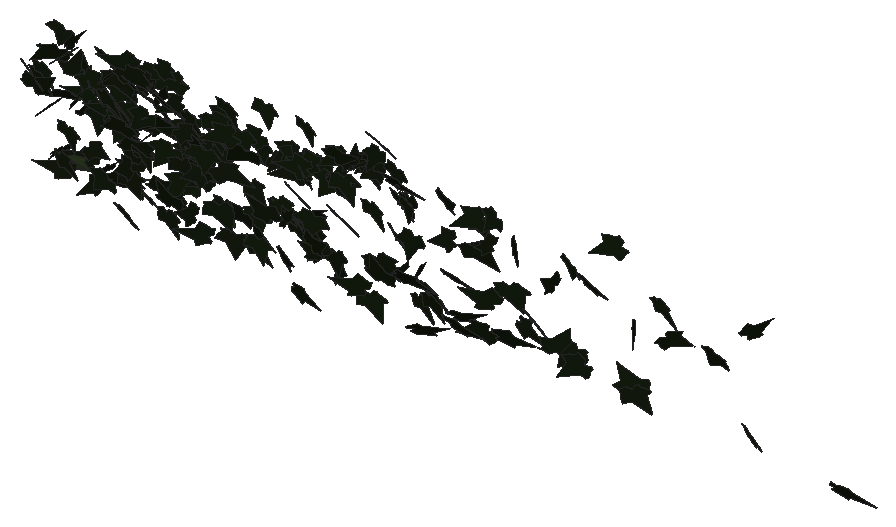
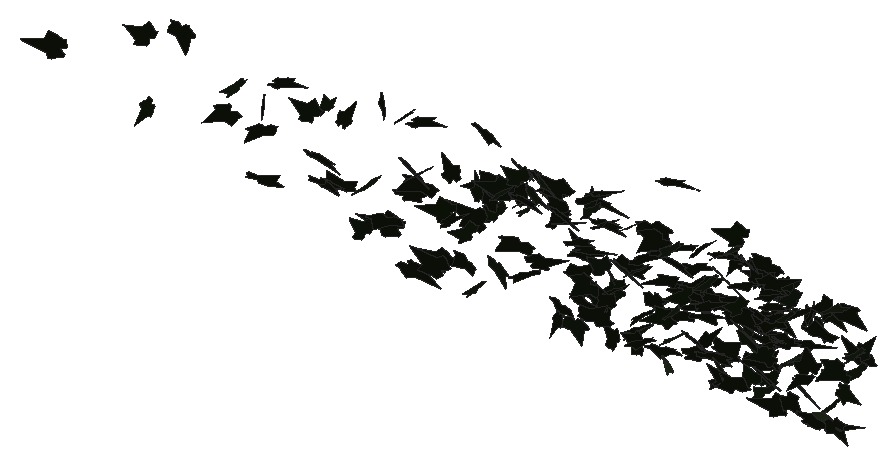
# SketchUp Ruby script. Lengths in millimetres.
U = 1.mm
M = Sketchup.active_model
def pt(a) = Geom::Point3d.new(a.map { |v| v * U })
def face(e, loops, mat)
  f = e.add_face(loops[0].map { |a| pt(a) })
  loops[1..].each { |l| e.add_face(l.map { |a| pt(a) }).erase! }
  f.material = f.back_material = mat if mat
  f
end
# faces: each face lists its corners as indices into pts; further lists are holes
def faces(e, pts, list, mat = nil) = list.each { |f| face(e, (f[0].is_a?(Array) ? f : [f]).map { |l| l.map { |i| pts[i] } }, mat) }
# xy, xz, yz: faces in a plane at the given z, y or x. An outline is a flat list of corners, or four numbers for a rectangle; further outlines are holes
def ring(l) = l.size == 4 ? [[l[0], l[1]], [l[2], l[1]], [l[2], l[3]], [l[0], l[3]]] : l.each_slice(2).to_a
def flat(e, list, mat, &to3) = list.each { |f| face(e, (f[0].is_a?(Array) ? f : [f]).map { |l| ring(l).map { |u, v| to3.(u, v) } }, mat) }
def xy(e, z, list, mat = nil) = flat(e, list, mat) { |x, y| [x, y, z] }
def xz(e, y, list, mat = nil) = flat(e, list, mat) { |x, z| [x, y, z] }
def yz(e, x, list, mat = nil) = flat(e, list, mat) { |y, z| [x, y, z] }
def lines(e, pts, list) = list.each { |a, b| e.add_line(pt(pts[a]), pt(pts[b])) }
# prism: a flat outline (further loops are holes) pulled along v
def prism(e, loops, v, mat = nil)
  f = face(e, loops, mat); d = Geom::Vector3d.new(v.map { |x| x * U })
  f.pushpull(f.normal.samedirection?(d) ? d.length : -d.length)
end
def box(e, o, s, mat = nil) = prism(e, [[o, [o[0] + s[0], o[1], o[2]], [o[0] + s[0], o[1] + s[1], o[2]], [o[0], o[1] + s[1], o[2]]]], [0, 0, s[2]], mat)
def at(x, y, z, deg = 0) = Geom::Transformation.translation(pt([x, y, z])) * Geom::Transformation.rotation(ORIGIN, Z_AXIS, deg.degrees)
def axes(o, x, y, z) = Geom::Transformation.new([*x, 0, *y, 0, *z, 0, *pt(o).to_a, 1])
def part(name) = M.definitions.add(name)
# library, detail: a bought-in or finely detailed component or shape, given as its bounding box
def library(name, o, s) = part(name).tap { |d| box(d.entities, o, s) }
def detail(e, o, s) = box(e.add_group.entities, o, s)
def put(e, d, t, mat = nil) = e.add_instance(d, t).tap { |i| i.material = mat if mat }
def group(e, t, mat = nil) = e.add_group.tap { |g| g.transformation = t; g.material = mat if mat }.entities
root = M.entities
M.materials.add("efeu1").color = [18, 25, 13]
M.materials.add("efeu2").color = [43, 57, 29]
c1 = part("ivyleaf_9")
p = [[39.1,54.8,31.7],[34.5,51.8,30.2],[-5.3,25.2,17.3],[-17.9,28.3,20.9],[-21.6,21.7,17],[-20.2,4.3,5.3],
  [-22.9,-0.3,2.5],[-17.1,-4,-0.6],[-2,-2.1,-1.2],[-0.7,-15.4,-10.1],[16.6,-22.3,-16.7],[21.1,-15.1,-12.5],
  [32.7,-10.7,-11],[46.1,-1.8,-6.6],[30.8,11.2,3.8]]
faces(c1.entities,p,[[0,1,2,3,4,5,6,7,8,9,10,11,12,13,14]],"efeu1")
c2 = part("ivyleaf_10")
p = [[0,12.8,-0.8],[-1.5,51.3,-10.9],[-4.9,51,-11.6],[-13.6,26.5,-7.3],[-13.2,15.9,-4.6],[-21.1,19.3,-7.2],
  [-29.5,16.3,-8.3],[-29.2,8.3,-6.2],[-19.7,-9.8,0.5],[-7.6,-13,4],[1,-12.2,5.8],[-0.4,51.1,-11.1],
  [-1.5,51.1,-10.9],[1,-12.4,5.9],[16.9,-12.4,3.5],[35.1,9.1,-5.1],[35,12.9,-6.1],[20.5,16.4,-4.9],
  [15.8,15,-3.8],[15.3,27.6,-7.1],[12.8,31.3,-7.8]]
faces(c2.entities,p,[[0,1,2,3,4,5,6,7,8,9,10],[11,12,0,13,14,15,16,17,18,19,20]],"efeu2")
put(root,c1,axes([8562.9,196.3,4759.8],[-2.19146,-0.0345,-0.92471],[1.76101,-0.06046,-1.14992],[-0.02091,-1.47557,0.06874]))
put(root,c1,axes([10984,192.4,4326.4],[1.98064,-0.46918,0.9956],[1.79725,-0.32316,-1.13939],[1.07594,1.4035,0.07047]))
put(root,c1,axes([8379.1,201,4482.6],[1.61589,-0.45567,1.0884],[-1.29664,0.90546,0.91054],[-1.83349,-1.04193,0.3153]))
put(root,c1,axes([8576.6,200,4294.5],[1.97099,0.92054,-0.5268],[0.75773,0.34504,1.38559],[1.87096,-1.10949,-0.00619]))
put(root,c1,axes([7499.4,228.5,4890.5],[-2.19386,-0.25774,0.753],[-1.3268,-0.31242,-1.17414],[0.73079,-1.34096,0.12883]))
put(root,c1,axes([7301.2,255.6,4612.9],[0.39628,-0.94646,-0.9854],[0.7097,-0.91957,0.96203],[-2.50164,-0.4108,0.11683]))
put(root,c1,axes([8467.4,219.5,4522],[2.4859,-0.15942,0.65079],[1.22484,-0.09825,-1.31575],[0.35484,1.45601,-0.01753]))
put(root,c1,axes([9769.6,253.2,4375.7],[-0.09431,-0.99216,-1.12416],[0.08743,1.12324,-0.99337],[2.85226,-0.06724,-0.00672]))
put(root,c1,axes([7837.6,274.7,4204.2],[0.73222,-0.0408,-1.35161],[2.5723,0.05563,0.38304],[0.08063,-1.4042,0.05445]))
put(root,c1,axes([10232,254.2,4723.3],[1.7276,0.08746,-1.15386],[-2.19146,-0.07716,-0.9117],[-0.21839,1.46609,0.02085]))
put(root,c1,axes([8038,300.5,4652.2],[1.28327,-1.06692,0.67998],[0.83341,-0.52609,-1.25968],[2.25907,0.80015,0.07845]))
put(root,c1,axes([9442,300.4,4373.5],[-2.8045,0.09058,-0.02],[0.038,-0.00121,-1.47635],[-0.1724,-1.47371,-0.00001]))
put(root,c1,axes([8499.3,305,4497.1],[0.61122,0.79492,1.08944],[-0.80571,-1.00387,0.85728],[2.43695,-0.53128,0.01019]))
put(root,c1,axes([7883.2,326.5,4423.3],[-0.31494,0.14937,1.40214],[1.07295,-1.28701,0.20364],[2.45984,0.5805,0.09069]))
put(root,c1,axes([8154.1,340.5,4291.7],[-0.59309,-0.05531,1.32072],[-2.4712,-0.24154,-0.31649],[0.47157,-1.33532,0.00254]))
put(root,c1,axes([6810.9,366.4,4422.7],[-0.38699,-0.39754,1.37191],[-1.16035,-1.229,-0.44649],[2.45834,-0.64268,0.00522]))
put(root,c1,axes([6675.7,376.5,4312.4],[-1.33984,-0.78621,1.05007],[-0.24028,-1.14559,-0.94237],[2.48499,-0.53467,0.47505]))
put(root,c1,axes([7811,365.8,4767.3],[-1.32302,0.07354,1.22552],[-1.98322,-0.78002,-0.54428],[1.23552,-1.17333,0.43864]))
put(root,c1,axes([8995.9,367.9,4811.6],[-0.2074,-0.10367,-1.49281],[2.55354,-0.66953,-0.05145],[-1.26106,-1.33869,0.14134]))
put(root,c1,axes([8190.7,361,4718.5],[0.6786,-1.36006,0.11868],[0.0953,-0.10955,-1.40587],[2.59656,0.35947,0.02058]))
put(root,c1,axes([6972.2,358,4845],[1.61148,-0.92304,0.76005],[1.12143,-0.48827,-1.24941],[1.98014,1.02772,0.08904]))
put(root,c1,axes([7808.5,379.1,4721.4],[-0.39822,-0.37855,1.33222],[-0.09954,-1.34422,-0.39017],[2.63397,-0.10803,0.18667]))
put(root,c1,axes([7803.3,362.4,4750.1],[-2.55961,0.24778,0.53086],[-1.01631,0.02819,-1.36602],[-0.45855,-1.4456,0.06436]))
put(root,c1,axes([6809.7,371.6,4164.1],[1.06727,-1.30141,0.24463],[-0.14908,0.2326,1.41695],[-2.5158,-0.56587,0.01981]))
put(root,c1,axes([10340.5,346.6,4327.8],[2.04102,-0.62296,-0.85036],[-1.3599,0.46226,-1.23976],[1.47499,1.28821,0.03366]))
put(root,c1,axes([7614.2,353.5,4460.5],[0.37473,0.0387,1.38181],[-2.04334,0.88348,0.12824],[-1.65722,-1.08057,0.15433]))
put(root,c1,axes([8334.9,345.6,4641.8],[1.37373,-0.04962,-1.16794],[-2.10127,0.42215,-0.70026],[0.73114,1.30647,0.18191]))
put(root,c1,axes([9209.5,385.3,4658.1],[0.35737,0.19372,1.43585],[-1.6555,-1.14281,0.26794],[2.2052,-0.88933,-0.03154]))
put(root,c1,axes([8174.9,375.5,4247.8],[-0.15432,-1.4151,-0.50641],[0.18079,0.50131,-1.41605],[2.85475,-0.10825,0.0623]))
put(root,c1,axes([7461.9,370.9,4736.7],[1.09678,0.60588,-1.21717],[-1.80986,-0.76522,-0.83115],[-1.8494,1.10817,0.09154]))
put(root,c1,axes([7880.1,390.2,4347.5],[0.45104,0.12332,1.3102],[-2.35687,-0.42955,0.26443],[0.84745,-1.26027,0.03808]))
put(root,c1,axes([9040.6,375.2,4410.1],[1.53966,-1.01172,-0.7666],[-0.52801,0.74614,-1.2775],[2.35742,0.82789,0.21454]))
put(root,c1,axes([7211.7,396.7,4633.1],[-1.24778,-1.16623,-0.35385],[0.27886,0.32346,-1.33756],[2.30267,-0.67114,-0.02977]))
put(root,c1,axes([9649.5,406.8,4601.4],[-0.30962,0.16582,-1.43387],[2.181,-0.86252,-0.22976],[-1.67033,-1.15695,-0.03422]))
put(root,c1,axes([7136.3,416.7,4271.7],[-0.13617,-0.07773,1.43345],[-1.72511,-1.1105,-0.10546],[2.11864,-0.90922,0.00626]))
put(root,c1,axes([8769.5,418,4829.5],[-1.90746,-0.64191,0.88595],[-1.41893,-0.47861,-1.19018],[1.52389,-1.24913,0.00074]))
put(root,c1,axes([7998.5,407.3,4768.2],[-0.2516,-1.43289,-0.42131],[0.11864,0.4173,-1.4388],[2.84004,-0.14437,0.02278]))
put(root,c1,axes([6636.1,405.3,4722.4],[1.31213,-1.28051,-0.16061],[-0.11086,0.15103,-1.45418],[2.45367,0.6916,0.02019]))
put(root,c1,axes([8835.3,410.7,4428.5],[-0.30373,0.12087,1.418],[-2.68691,-0.19332,-0.14241],[0.34144,-1.41379,0.1407]))
put(root,c1,axes([7089.9,402.7,4537.9],[-0.98167,-0.64825,-1.06719],[1.39495,0.77762,-0.8266],[1.92394,-0.89457,0.05481]))
put(root,c1,axes([7208.2,420,4192],[-0.88373,-0.17301,1.28913],[-2.32953,-0.40492,-0.49522],[0.83741,-1.30901,-0.01719]))
put(root,c1,axes([6679.1,425,4690.5],[0.69508,-0.8913,1.08843],[0.66825,-1.03117,-0.96222],[2.59269,0.50473,-0.04379]))
put(root,c1,axes([7818.8,426.4,4497.5],[-1.6403,-1.09961,-0.07568],[0.09317,0.05778,-1.39712],[2.09565,-0.86325,0.00288]))
put(root,c1,axes([6983,423.6,4227.5],[0.47095,-1.41829,0.05295],[0.02191,-0.05175,-1.43971],[2.70108,0.24771,0.00244]))
put(root,c1,axes([7290.7,411.5,4375.3],[-1.10468,-0.88967,-0.93929],[0.92443,0.80432,-1.06199],[2.28213,-0.75646,-0.02449]))
put(root,c1,axes([7814.7,429.6,4766.3],[-1.1039,0.03341,1.20078],[-1.88632,-0.76671,-0.45742],[1.29172,-1.09108,0.3582]))
put(root,c1,axes([6995.7,429.3,4557.6],[-2.02387,-0.86123,0.10606],[-0.14921,-0.07171,-1.3684],[1.64472,-1.06627,0.00637]))
put(root,c1,axes([7430.1,400.6,4396.3],[0.96745,0.08596,-1.26753],[-2.40719,-0.09413,-0.51362],[-0.22736,1.36241,0.04449]))
put(root,c1,axes([8457.2,423.3,4370.7],[1.4704,-1.23284,0.36713],[0.45249,-0.28402,-1.4541],[2.406,0.80686,0.0491]))
put(root,c1,axes([6603.6,412.1,4250.4],[-2.23352,0.87514,-0.27672],[0.42885,-0.16072,-1.46393],[-1.6934,-1.19498,-0.00576]))
put(root,c1,axes([9219.5,399.4,4325.2],[-1.78036,-0.22029,1.16347],[2.16538,0.24373,0.96092],[-0.6246,1.47287,0.015]))
put(root,c1,axes([9303.3,427.3,4346.9],[-2.56536,-0.42922,-0.17601],[0.32265,0.0477,-1.4146],[0.82183,-1.35853,0.00594]))
put(root,c1,axes([7394.4,399.1,4704.7],[2.41644,0.4718,0.15703],[0.27625,0.06021,-1.35448],[-0.90515,1.27793,0.00584]))
put(root,c1,axes([8826.8,451.3,4839.4],[-0.67327,-0.93984,0.94769],[-0.6534,-0.88335,-1.00419],[2.45472,-0.49291,-0.00737]))
put(root,c1,axes([7218.7,427.4,4484.3],[0.95034,0.07886,1.25223],[-2.3413,0.29591,0.47191],[-0.46977,-1.31524,0.18126]))
put(root,c1,axes([6759,435,4335],[-1.09066,-0.43894,-1.08951],[2.08874,0.23193,-0.6707],[0.79668,-1.20899,0.26689]))
put(root,c1,axes([8182.2,421.1,4420.7],[-0.61876,-0.49084,-1.27348],[1.43092,1.02815,-0.58822],[2.16781,-0.81876,0.02478]))
put(root,c1,axes([6791.6,421.8,4482.3],[-0.52047,-0.1721,1.42562],[2.72064,-0.17012,0.25368],[0.25893,1.4416,0.20012]))
put(root,c1,axes([9249.7,458.2,4742.1],[-0.15948,-0.86519,1.12515],[0.15552,-1.12818,-0.86143],[2.6968,0.01389,0.11622]))
put(root,c1,axes([7675.9,405,4438.8],[-0.157,0.66584,1.14036],[-0.17119,1.13709,-0.67044],[-2.50736,-0.11932,-0.02563]))
put(root,c1,axes([7930.3,441.3,4684.5],[-0.43372,0.30578,1.36223],[1.24837,-1.19499,0.37797],[2.3456,0.69254,0.05072]))
put(root,c1,axes([8875.7,434,4257.6],[1.42113,-0.22488,1.26706],[2.31834,-0.34884,-0.77978],[0.78972,1.42875,0.00904]))
put(root,c1,axes([6998.5,433.7,4277.5],[1.18369,-0.51307,1.18328],[-1.34624,0.96277,0.78926],[-2.05249,-0.92738,0.16473]))
put(root,c1,axes([7477.1,452.9,4247.9],[-0.34424,-1.35009,-0.11912],[0.02933,0.11812,-1.36215],[2.57931,-0.18153,-0.00041]))
put(root,c1,axes([6810.4,459.6,4488.8],[0.2379,-1.4241,0.3036],[0.09461,-0.30037,-1.4294],[2.76964,0.13259,0.02275]))
put(root,c1,axes([9327.9,459.2,4686.5],[0.81993,-0.81644,1.17668],[1.27057,-0.97262,-0.91928],[2.41148,0.79006,0.08427]))
put(root,c1,axes([6724.8,438.4,4575.6],[0.29554,0.25106,-1.28978],[-2.23841,-0.55256,-0.24916],[-1.11511,1.17573,0.15832]))
put(root,c1,axes([7451.2,445.1,4236.9],[1.09645,-1.23103,-0.41821],[-0.09266,0.43668,-1.35247],[2.47267,0.56224,0.13476]))
put(root,c1,axes([8560.3,450.9,4455],[1.94534,-0.71119,0.69823],[1.29846,-0.22979,-1.23281],[1.38274,1.21634,0.17535]))
put(root,c1,axes([7273.7,439,4551.9],[0.67511,-0.54715,-1.30549],[1.09818,1.28486,-0.38172],[2.46002,-0.42342,0.52867]))
put(root,c1,axes([6373.5,476.6,4422.8],[0.2091,-1.33462,0.44618],[0.11601,-0.44261,-1.33893],[2.67572,0.12348,0.02318]))
put(root,c1,axes([9633.8,455.6,4247.2],[-2.74587,-0.45103,-0.0833],[-0.12569,-0.0678,1.51095],[-0.86382,1.44358,0.04494]))
put(root,c1,axes([8572.4,470.8,4197.4],[1.12034,-0.67747,1.19795],[1.87713,-0.70102,-0.8811],[1.82673,1.13586,0.17071]))
put(root,c1,axes([6723.9,473.4,4777.3],[1.58294,-0.8329,0.70912],[0.98386,-0.48579,-1.17691],[1.83473,0.9791,0.0193]))
put(root,c1,axes([6443.4,435.3,4596.8],[0.48885,0.43655,1.37704],[0.71484,1.33035,-0.49181],[-2.65477,0.43861,0.12114]))
put(root,c1,axes([6722.5,462.8,4841.8],[0.04039,-0.30515,-1.37922],[2.05175,0.89482,-0.18139],[1.7372,-1.04975,0.2463]))
put(root,c1,axes([7326.6,477.3,4210],[-1.64389,-0.86096,-0.59236],[0.86775,0.38105,-1.21866],[1.78967,-0.97558,0.04677]))
put(root,c1,axes([6921.1,441.8,4799.6],[-0.07471,0.02081,-1.39293],[-1.45993,1.16288,0.03899],[2.21318,0.7678,-0.0213]))
put(root,c1,axes([7658.1,496.2,4726.9],[-1.31772,-0.92516,0.77717],[-0.76214,-0.6694,-1.15362],[2.16961,-0.79705,0.06677]))
put(root,c1,axes([6339,474.6,4268.3],[1.13354,-1.14201,-0.35397],[-0.34258,0.30531,-1.28787],[2.24955,0.62195,-0.01776]))
put(root,c1,axes([6795.7,496.8,4230.2],[-0.28172,-0.73805,1.18023],[0.81543,-1.15342,-0.66755],[2.52064,0.29064,0.34786]))
put(root,c1,axes([7033.5,456.5,4655.9],[0.74188,-0.4459,-1.19635],[-0.23245,1.2321,-0.49902],[2.41875,0.25517,0.31899]))
put(root,c1,axes([7201.3,475.3,4771.6],[0.12231,-1.04309,-0.8488],[0.61125,0.83708,-1.00438],[2.48537,-0.15454,0.28879]))
put(root,c1,axes([10265.5,457,4749.5],[0.04717,-0.28257,1.49077],[2.36273,0.861,0.14256],[-1.6603,1.21724,0.24523]))
put(root,c1,axes([7859.2,504.6,4670.2],[-1.70968,-0.97027,0.43051],[0.0091,-0.56767,-1.26943],[2.02021,-0.81857,0.37005]))
put(root,c1,axes([7896,482.5,4803.5],[0.1617,-0.10711,1.45815],[2.45717,-0.67996,-0.12518],[1.30587,1.2927,0.05498]))
put(root,c1,axes([9723,493.4,4702.1],[1.20597,-1.35624,0.03576],[0.00494,-0.03825,-1.4969],[2.58209,0.63351,-0.01383]))
put(root,c1,axes([6823.9,491.8,4823],[-2.22161,0.35084,-0.54823],[0.92732,-0.27538,-1.21367],[-0.82134,-1.25989,0.11262]))
put(root,c1,axes([6571.9,491.7,4644.3],[1.10354,-1.22517,-0.08795],[-0.07145,0.07954,-1.35545],[2.33665,0.58105,0.00009]))
put(root,c1,axes([8426.3,491.5,4273.9],[-0.88135,-0.00804,-1.29447],[2.45034,0.13998,-0.46146],[0.25597,-1.36766,-0.03962]))
put(root,c1,axes([7659.1,497.8,4746.9],[-2.57946,-0.27286,0.18589],[-0.34009,-0.05418,-1.38241],[0.52838,-1.36694,0.01768]))
put(root,c1,axes([7116.6,495.9,4561.1],[1.80331,-0.72708,0.58664],[-0.74777,0.44794,1.18977],[-1.61315,-1.02043,0.10428]))
put(root,c1,axes([6171.8,492,4558.1],[-0.98579,0.33562,1.261],[1.83286,-0.81715,0.61307],[1.67579,1.09117,0.07126]))
put(root,c1,axes([6596,461.2,4760.5],[0.72814,0.88871,1.07059],[0.81351,0.98156,-0.96756],[-2.52005,0.57365,-0.00301]))
put(root,c1,axes([6287.9,503.7,4781.9],[0.2609,0.50986,-1.36194],[-0.92348,-1.27355,-0.52561],[-2.60912,0.50175,0.04985]))
put(root,c1,axes([7561,514,4179.8],[1.4102,-0.60878,-1.0482],[2.01664,-0.27136,0.90663],[-1.12044,-1.25464,0.31252]))
put(root,c1,axes([6168.5,503,4588.9],[0.88986,-1.25664,0.56074],[-0.144,0.56785,1.33566],[-2.61497,-0.4589,0.11726]))
put(root,c1,axes([7999,466.6,4819.2],[-1.67494,0.88712,-0.84277],[-1.11682,0.60496,1.24957],[2.04353,1.05773,-0.00785]))
put(root,c1,axes([7625.8,516.2,4525.3],[0.67725,-0.86092,0.90075],[0.83209,-0.79093,-0.92868],[2.22062,0.55894,0.07327]))
put(root,c1,axes([7713,507.6,4384.1],[1.38483,-1.21166,0.00874],[0.00234,-0.00945,-1.41335],[2.30609,0.72762,-0.00381]))
put(root,c1,axes([7330.5,515.1,4712.9],[-0.5517,-1.37156,-0.16549],[0.02622,0.16622,-1.40171],[2.62916,-0.28947,-0.02075]))
put(root,c1,axes([6677.2,514.8,4533.5],[-2.14984,-0.61964,-0.2132],[0.40085,0.05904,-1.28746],[1.18099,-1.14802,0.04887]))
put(root,c1,axes([7541.7,503.4,4440.9],[2.22382,-0.88159,0.07129],[0.12694,-0.02996,-1.46364],[1.67853,1.17025,0.01624]))
put(root,c1,axes([6450.5,529.9,4668.1],[-0.06413,-0.40846,1.28253],[-0.02682,-1.28275,-0.4089],[2.56157,-0.02366,0.02783]))
put(root,c1,axes([9783.2,478.9,4553],[0.04762,0.07779,-1.48039],[-0.08883,1.47991,0.07698],[2.81997,0.0453,0.02743]))
put(root,c1,axes([6495,487.1,4361.8],[0.42354,-0.38761,-1.20915],[-0.52692,1.18323,-0.43026],[2.35846,0.33396,0.12102]))
put(root,c1,axes([6745.5,526.2,4764.8],[-0.37616,0.10804,1.41294],[0.41715,-1.40711,0.13826],[2.66449,0.23555,0.17783]))
put(root,c1,axes([6465.1,499.7,4715.3],[0.72629,-0.96952,-0.97267],[0.07954,1.01726,-0.99756],[2.61253,0.23856,0.30078]))
put(root,c1,axes([6787.4,519.4,4615.3],[-2.41877,-0.07683,-0.32492],[0.62883,-0.10552,-1.26742],[0.09138,-1.30752,0.12137]))
put(root,c1,axes([6333,522.3,4175.1],[-1.00012,0.03406,1.28189],[-2.39828,-0.27044,-0.50939],[0.45226,-1.35877,0.13352]))
put(root,c1,axes([6629.3,513.1,4767.1],[-1.04254,-0.65832,-1.24387],[1.92442,0.74429,-0.83921],[1.86298,-1.13724,0.17081]))
put(root,c1,axes([7548.3,512.1,4447.1],[0.48633,-1.25168,-0.58974],[0.07126,0.60575,-1.26943],[2.63241,0.21485,0.14332]))
put(root,c1,axes([8760.3,499.4,4653.9],[-1.56124,1.07741,0.37079],[-0.44807,0.28676,-1.35409],[-2.12176,-0.85334,0.01312]))
put(root,c1,axes([8098.9,524.2,4886.2],[-2.11632,0.14756,-0.71953],[1.32327,-0.20943,-1.11746],[-0.45069,-1.30781,0.09776]))
put(root,c1,axes([6960.7,532.5,4839.6],[-2.28307,-0.27111,0.6453],[-1.04669,-0.42696,-1.20174],[0.82401,-1.2935,0.26142]))
put(root,c1,axes([7111,536.2,4523.4],[-1.87247,-0.80675,0.37955],[-0.52368,-0.26289,-1.27202],[1.61401,-1.02123,0.02761]))
put(root,c1,axes([7217,534.9,4316.2],[0.0365,-1.29717,0.25437],[0.17622,-0.25246,-1.29438],[2.50962,0.03659,0.08719]))
put(root,c1,axes([7029.2,519.7,4588.7],[-0.90353,-0.14858,-1.35587],[-2.33843,-0.57682,0.49342],[-1.12723,1.31569,0.06321]))
put(root,c1,axes([7892,505.9,4662.5],[-0.99366,-0.67272,1.24259],[1.65156,0.8928,0.84796],[-2.12234,1.00972,0.07809]))
put(root,c1,axes([6967.8,521.8,4740.1],[-2.24175,0.74236,-0.13039],[0.21108,-0.06857,-1.3923],[-1.41887,-1.1831,-0.00112]))
put(root,c1,axes([8651.8,516.1,4600.2],[-0.64704,-0.2818,-1.39283],[1.82793,1.00994,-0.43877],[1.99329,-1.01763,-0.04976]))
put(root,c1,axes([7399.6,538.6,4230.7],[0.8948,-0.15022,-1.34261],[2.51632,-0.24099,0.48995],[-0.5284,-1.40199,0.05964]))
put(root,c1,axes([8262,538,4700.9],[-1.48073,0.08206,-1.19661],[2.22733,-0.26042,-0.77878],[-0.49991,-1.40334,0.07455]))
put(root,c1,axes([6340,529.8,4775.9],[-1.00516,1.0432,-0.71727],[0.27941,-0.72147,-1.15741],[-2.39318,-0.52239,0.16613]))
put(root,c1,axes([7847,537.8,4273.2],[-1.56117,-0.06383,-1.01081],[1.92014,0.06287,-0.82271],[0.16949,-1.30025,0.00984]))
put(root,c1,axes([6628.3,534.3,4587.8],[0.82743,-1.18671,-0.32652],[-0.16308,0.31627,-1.26355],[2.33681,0.44227,0.02744]))
put(root,c1,axes([6437.5,527.8,4693.8],[-0.27732,-1.0684,0.82613],[1.0188,0.71717,1.02191],[-2.35983,0.43518,0.3441]))
put(root,c1,axes([8234.8,508.8,4327.1],[-0.42045,1.30626,0.52084],[-0.15359,0.51458,-1.3248],[-2.672,-0.23512,-0.00581]))
put(root,c1,axes([6613,556.8,4670.6],[-1.01854,-1.04783,0.62057],[-0.24802,-0.62468,-1.16716],[2.30442,-0.53037,0.14867]))
put(root,c1,axes([7603.8,539.9,4347.8],[1.16927,-1.24201,-0.09434],[-0.06035,0.08956,-1.3856],[2.36982,0.61508,0.01126]))
put(root,c1,axes([8545.4,528.5,4208.2],[2.17589,0.76944,-0.3911],[0.61992,0.21648,1.37809],[1.52125,-1.18877,-0.00219]))
put(root,c1,axes([7036.3,552.7,4511.8],[-2.00047,-0.93043,0.08005],[-0.09587,-0.06385,-1.40368],[1.77475,-1.05222,0.0144]))
put(root,c1,axes([6864.5,524.2,4893.2],[1.59044,-0.82721,-0.74649],[-0.22898,0.86066,-1.08841],[2.10822,0.71753,0.44493]))
put(root,c1,axes([6732.4,547.1,4362.5],[0.90381,0.17671,1.32123],[-2.51113,-0.1373,0.4926],[0.36106,-1.39725,0.11869]))
put(root,c1,axes([6674.1,557.9,4241.4],[0.28019,-1.23578,0.57859],[0.49556,-0.54581,-1.23203],[2.54924,0.24193,0.17591]))
put(root,c1,axes([6968.9,509.1,4256.6],[-0.11236,0.80555,1.17536],[-0.06107,1.17531,-0.80714],[-2.71121,-0.05986,-0.03053]))
put(root,c1,axes([6995.1,543.1,4681.3],[1.22481,-1.1734,-0.1858],[-0.12749,0.17513,-1.33806],[2.25744,0.64654,0.02524]))
put(root,c1,axes([6480,562.1,4492.8],[-0.32186,-1.2391,0.56615],[-0.07509,-0.5658,-1.25012],[2.59166,-0.17028,0.03409]))
put(root,c1,axes([6997.4,559.3,4328.6],[-2.49461,-0.66381,0.23282],[-0.35525,-0.14648,-1.46854],[1.29082,-1.32318,0.04578]))
put(root,c1,axes([6840,549.1,4595.2],[-0.02445,0.72202,-1.1828],[-0.49613,-1.163,-0.7071],[-2.5903,0.21594,0.1466]))
put(root,c1,axes([9441.5,564.8,4857.5],[-1.74702,-0.61078,0.9107],[-1.49738,-0.46044,-1.10182],[1.4537,-1.2083,-0.04048]))
put(root,c1,axes([6548.5,547.4,4258.5],[-0.6023,0.92222,-0.85565],[0.56275,-0.80306,-0.97491],[-2.3272,-0.43287,-0.01429]))
put(root,c1,axes([6731.1,527.2,4314.1],[-1.01871,0.82685,0.88023],[-1.07075,0.68123,-0.98203],[-2.03381,-0.77281,0.07612]))
put(root,c1,axes([6657.6,559,4804.2],[-0.51991,0.00404,1.42058],[-2.61331,-0.3716,-0.26299],[0.6931,-1.39806,0.07401]))
put(root,c1,axes([6640.5,552.7,4606.3],[-0.74664,-1.14408,-0.54111],[0.37299,0.50476,-1.20931],[2.37962,-0.43809,0.01977]))
put(root,c1,axes([8309.9,556.5,4200.5],[0.91709,-1.31411,-0.02725],[-0.04412,0.02052,-1.39959],[2.50116,0.4822,-0.0147]))
put(root,c1,axes([8699.2,549.7,4177.8],[0.09898,0.08608,-1.43616],[-2.19491,-0.85671,-0.09311],[-1.6371,1.15382,0.03801]))
put(root,c1,axes([8149.8,552.1,4747.6],[1.70844,-0.69292,0.9461],[1.58894,-0.4591,-1.12838],[1.56736,1.22071,0.11266]))
put(root,c1,axes([6602.9,559.8,4525.9],[-0.6507,-1.28681,-0.31378],[0.20481,0.29601,-1.33118],[2.51248,-0.3574,0.02725]))
put(root,c1,axes([7182.3,565.6,4553],[0.01171,-1.28315,0.20176],[0.03428,-0.20166,-1.28306],[2.47186,0.00888,0.01684]))
put(root,c1,axes([7559.4,569.5,4383.5],[-0.05099,-0.37717,1.31538],[0.83279,-1.24892,-0.3492],[2.46758,0.41371,0.14503]))
put(root,c1,axes([6594.4,562.2,4538],[-0.95318,-0.07317,1.26982],[-2.40404,-0.13137,-0.50577],[0.28377,-1.35868,-0.01948]))
put(root,c1,axes([7870.5,527.8,4199.8],[0.25738,-0.16457,-1.37499],[-1.65174,1.06649,-0.21301],[2.05377,0.87835,0.00101]))
put(root,c1,axes([8254.2,536.3,4681.9],[1.14193,-0.09941,-1.27835],[-2.37878,0.26958,-0.60761],[0.5445,1.38619,0.02648]))
put(root,c1,axes([8440.1,572.2,4731.8],[-0.28984,-0.16631,1.41236],[0.76711,-1.36724,-0.11753],[2.59559,0.38551,0.19245]))
put(root,c1,axes([7123.3,556.2,4597.6],[-1.18941,-0.85754,-0.91346],[1.15695,0.68505,-1.05901],[2.08505,-0.8693,0.06654]))
put(root,c1,axes([7196.6,571.1,4789.2],[0.45876,-1.26746,0.4019],[0.26029,-0.38265,-1.28878],[2.51718,0.27057,0.06002]))
put(root,c1,axes([7694.8,528.2,4428.8],[1.5103,0.92156,0.60672],[0.75084,0.46094,-1.21614],[-1.96107,0.88621,0.00163]))
put(root,c2,axes([6337.7,545.3,4223],[-1.60892,-0.26673,-0.90688],[1.63555,0.28995,-0.88637],[0.74943,-1.20542,-0.01254]))
put(root,c1,axes([6791.2,553.9,4510.6],[-0.99169,1.15113,-0.56608],[0.46523,-0.5107,-1.26352],[-2.39666,-0.57545,-0.01104]))
put(root,c1,axes([7113.9,556,4383.5],[-2.16236,0.55762,0.10034],[-0.15109,0.06594,-1.2654],[-1.06767,-1.13868,-0.02415]))
put(root,c1,axes([8005,563.1,4807.4],[-1.77661,0.69519,-0.62259],[0.7176,-0.52456,-1.15107],[-1.62469,-0.99189,0.17239]))
put(root,c1,axes([6145.3,569.3,4625.4],[0.68491,-1.27124,0.13204],[0.09557,-0.123,-1.32111],[2.43055,0.36306,0.01474]))
put(root,c1,axes([7374.6,582.6,4692],[-0.00893,-0.8214,-1.09659],[-0.03503,-1.09646,0.82139],[-2.60736,0.01754,-0.00728]))
put(root,c1,axes([6448.5,567.9,4574.9],[-1.34539,0.2319,1.06224],[-2.0444,-0.34484,-0.63958],[0.3199,-1.22848,0.38005]))
put(root,c1,axes([7722.5,544.5,4313.1],[-0.21426,0.1104,1.3975],[-1.75272,1.05121,-0.15723],[-2.01153,-0.92771,-0.01186]))
put(root,c1,axes([8039.5,590.1,4741.1],[-1.12297,-0.63206,1.05251],[-0.70039,-1.023,-0.82065],[2.22914,-0.63983,0.27237]))
put(root,c1,axes([7206.8,570,4741.3],[-2.48109,0.13098,0.02587],[-0.05043,-0.0049,-1.31018],[-0.24904,-1.30389,0.00753]))
put(root,c1,axes([6666.1,575.3,4539.7],[-2.08936,-0.66312,-0.22872],[0.33034,0.15478,-1.28186],[1.2935,-1.11065,-0.04208]))
put(root,c1,axes([7860.5,568.4,4763.1],[-2.49718,0.36922,-0.01084],[0.01965,-0.0033,-1.36306],[-0.70273,-1.31214,0.00038]))
put(root,c1,axes([6908.9,580.7,4229],[0.59844,-1.17906,0.32507],[0.17535,-0.31185,-1.22024],[2.32109,0.32755,0.00837]))
put(root,c1,axes([7635.1,586.6,4837.9],[0.30313,-1.22228,0.55434],[0.15285,-0.54855,-1.23259],[2.54973,0.1782,0.00799]))
put(root,c1,axes([6637.5,563.3,4450.3],[2.24835,-0.44659,0.29333],[0.50174,-0.13193,-1.26261],[0.88448,1.21006,-0.0294]))
put(root,c1,axes([7756.4,552.9,4224],[0.18639,1.27164,-0.20626],[-0.04142,-0.20519,-1.27539],[-2.45146,0.10015,0.00587]))
put(root,c2,axes([7222.6,572.3,4216.4],[1.65363,-0.88769,0.20514],[0.45934,-0.04909,-1.23465],[1.67204,0.89141,0.1363]))
put(root,c1,axes([7215.2,560.9,4438],[2.26623,-0.32832,0.32068],[0.66417,0.06861,-1.22557],[0.56728,1.23126,0.15381]))
put(root,c1,axes([6793.9,581.3,4645.1],[1.24185,-1.08366,0.47657],[0.49069,-0.40103,-1.26488],[2.19898,0.70147,0.01311]))
put(root,c1,axes([7407.2,587.9,4851.1],[-0.21424,-1.34264,0.15888],[0.03049,-0.16074,-1.34704],[2.57297,-0.10989,0.02919]))
put(root,c1,axes([6577.1,553.4,4200.5],[0.9033,0.09126,1.31483],[2.44319,0.28459,-0.48315],[-0.56827,1.3686,0.01279]))
put(root,c1,axes([8167.6,593.1,4647.7],[0.68264,-1.21953,0.74235],[0.46858,-0.70112,-1.27075],[2.6765,0.43379,0.03314]))
put(root,c1,axes([8920,595.4,4290.6],[0.55397,-0.96746,1.08973],[0.74484,-1.01853,-1.00878],[2.67149,0.48459,0.05529]))
put(root,c1,axes([7500.8,563.3,4606.6],[-1.4519,0.98086,0.37583],[-0.6987,0.18622,-1.2312],[-1.87304,-0.82979,0.16795]))
put(root,c1,axes([6479.1,584.8,4797.1],[1.38799,-1.09657,0.29524],[0.3124,-0.24541,-1.31695],[2.13862,0.74754,0.00076]))
put(root,c1,axes([6253.9,602.3,4825.7],[-1.18191,-1.01482,0.65794],[0.35566,-0.81124,-1.07488],[2.27416,-0.40054,0.51004]))
put(root,c1,axes([6400.5,582.3,4469.8],[1.52841,0.71394,0.80886],[-1.18339,-0.51775,1.07434],[1.67799,-1.01544,0.02092]))
put(root,c1,axes([7728.1,596.7,4663.4],[-1.75209,-0.80956,0.49178],[-0.72018,-0.31436,-1.22586],[1.65265,-0.99526,-0.01283]))
put(root,c1,axes([6265.5,574.6,4241.9],[-0.418,1.09343,-0.60107],[0.23966,-0.58777,-1.11525],[-2.36259,-0.25308,-0.00679]))
put(root,c1,axes([6626.5,596.8,4718.4],[-1.83407,-0.44899,0.76497],[-1.2467,-0.40136,-1.06078],[1.13823,-1.16308,0.07075]))
put(root,c1,axes([6318.5,551,4795.7],[0.24744,0.21997,1.39178],[1.52652,1.1376,-0.25472],[-2.20486,0.8123,-0.02016]))
put(root,c1,axes([7169,607.5,4487.9],[-0.59856,-0.86879,0.98752],[-0.31729,-0.98083,-0.91601],[2.48307,-0.33476,0.121]))
put(root,c1,axes([6837.1,575.2,4223.8],[-0.83106,0.01491,1.42325],[2.59604,-0.42083,0.42291],[0.77373,1.42802,0.10977]))
put(root,c1,axes([7354.5,593.1,4284.3],[-0.56338,-1.32053,-0.25073],[0.03976,0.25219,-1.35287],[2.55782,-0.29478,-0.0342]))
put(root,c1,axes([6620.3,597.2,4775.6],[-0.91707,-1.22323,-0.06714],[0.16876,0.03714,-1.31292],[2.32545,-0.48509,0.0688]))
put(root,c1,axes([6823.2,574.5,4548.3],[-1.76564,0.93372,0.23511],[-0.35206,0.14757,-1.31597],[-1.79838,-0.9456,0.02679]))
put(root,c1,axes([6354,573,4658.2],[-2.32295,0.16301,0.61936],[1.11933,-0.2424,1.22281],[0.48252,1.34706,0.1451]))
put(root,c1,axes([8602.6,584.5,4704.6],[0.73519,-1.30055,-0.54488],[-0.10093,0.55115,-1.35313],[2.68176,0.37728,0.09845]))
put(root,c1,axes([7336.3,583.1,4427.8],[0.50658,-1.17217,-0.62284],[-0.28958,0.60411,-1.20195],[2.50961,0.30632,-0.01297]))
put(root,c1,axes([6102.1,594.7,4568.1],[0.99971,-1.19343,0.18934],[0.14958,-0.17227,-1.30391],[2.29488,0.53112,0.00251]))
put(root,c1,axes([6993.6,604.6,4588.6],[-0.94452,-0.03954,1.22679],[-2.00408,-0.6662,-0.44745],[1.20029,-1.14345,0.21827]))
put(root,c1,axes([6412.5,585.2,4212.9],[-1.21991,0.25346,1.19319],[-2.11181,0.43871,-0.68927],[-0.96428,-1.28144,0.00003]))
put(root,c1,axes([6230.8,564.1,4518.5],[2.05809,0.65846,0.54013],[0.80417,0.34315,-1.26428],[-1.40731,1.15904,0.06746]))
put(root,c1,axes([7365.8,608.1,4641],[-0.14968,-1.28965,0.34276],[0.1174,-0.3465,-1.28957],[2.53696,-0.06005,0.0799]))
put(root,c1,axes([6203.3,600.6,4443],[-1.20018,0.58043,-0.95952],[0.70075,-0.93264,-0.80615],[-2.01597,-0.66974,0.29103]))
put(root,c1,axes([7976.2,599.8,4744.8],[0.71172,-1.26073,-0.04138],[-0.00598,0.04223,-1.31499],[2.40071,0.37387,0.00899]))
put(root,c1,axes([7613.9,597.1,4305.2],[1.51546,-0.16263,1.10794],[-2.05381,0.25165,0.8125],[-0.5692,-1.34099,0.01811]))
put(root,c1,axes([8442.2,616.6,4517.4],[-0.73888,-0.39136,1.26453],[-1.5916,-0.94899,-0.55046],[1.95285,-0.92152,0.02982]))
put(root,c1,axes([7086.5,596.2,4607.6],[1.90554,-1.01155,0.16192],[0.20018,-0.12371,-1.42321],[1.93938,1.00667,-0.01219]))
put(root,c1,axes([8132.1,616.7,4765.8],[-0.24933,-1.18829,0.66611],[0.01905,-0.67,-1.19327],[2.59256,-0.10936,0.07283]))
put(root,c1,axes([8022.5,610.4,4880.7],[0.58655,-0.96206,0.9269],[1.15103,-0.74771,-0.97716],[2.26707,0.62853,0.25631]))
put(root,c1,axes([7672.7,606.9,4643.2],[-1.54592,0.08622,1.0327],[-1.92174,-0.36095,-0.76408],[0.44357,-1.26331,0.28879]))
put(root,c1,axes([8035.7,605,4782.1],[-2.50851,-0.07378,0.01667],[-0.02401,-0.07241,-1.31817],[0.14194,-1.31617,0.07158]))
put(root,c1,axes([8794.6,597.2,4409.3],[-0.97312,-0.98332,-0.98037],[0.86152,0.86961,-1.10831],[2.4983,-0.68289,0.00032]))
put(root,c1,axes([6762.9,614.3,4791.6],[-1.31775,-1.12487,0.0702],[-0.06722,-0.06069,-1.32088],[2.14397,-0.69328,0.00173]))
